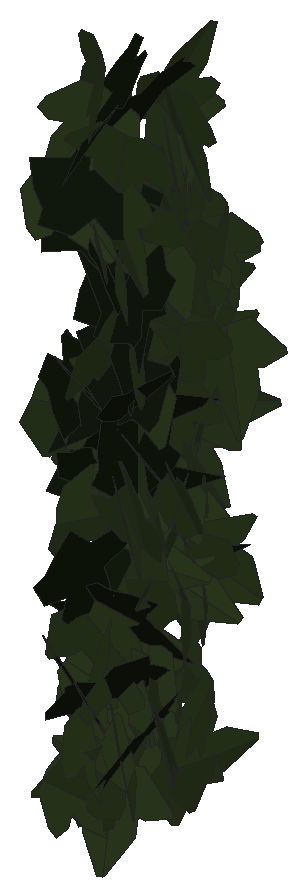
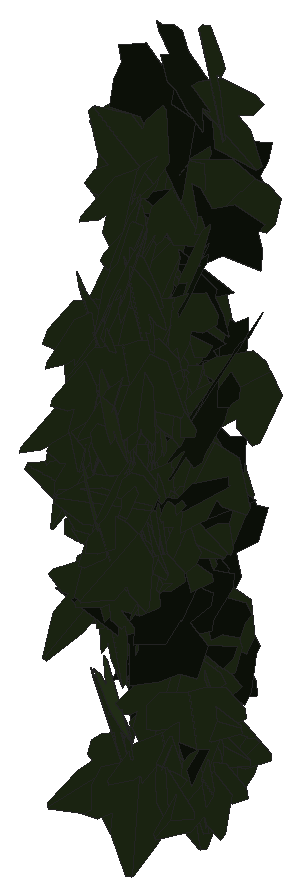
# SketchUp Ruby script. Lengths in inches.
U = 1.inch
M = Sketchup.active_model
def pt(a) = Geom::Point3d.new(a.map { |v| v * U })
def face(e, loops, mat)
  f = e.add_face(loops[0].map { |a| pt(a) })
  loops[1..].each { |l| e.add_face(l.map { |a| pt(a) }).erase! }
  f.material = f.back_material = mat if mat
  f
end
# faces: each face lists its corners as indices into pts; further lists are holes
def faces(e, pts, list, mat = nil) = list.each { |f| face(e, (f[0].is_a?(Array) ? f : [f]).map { |l| l.map { |i| pts[i] } }, mat) }
# xy, xz, yz: faces in a plane at the given z, y or x. An outline is a flat list of corners, or four numbers for a rectangle; further outlines are holes
def ring(l) = l.size == 4 ? [[l[0], l[1]], [l[2], l[1]], [l[2], l[3]], [l[0], l[3]]] : l.each_slice(2).to_a
def flat(e, list, mat, &to3) = list.each { |f| face(e, (f[0].is_a?(Array) ? f : [f]).map { |l| ring(l).map { |u, v| to3.(u, v) } }, mat) }
def xy(e, z, list, mat = nil) = flat(e, list, mat) { |x, y| [x, y, z] }
def xz(e, y, list, mat = nil) = flat(e, list, mat) { |x, z| [x, y, z] }
def yz(e, x, list, mat = nil) = flat(e, list, mat) { |y, z| [x, y, z] }
def lines(e, pts, list) = list.each { |a, b| e.add_line(pt(pts[a]), pt(pts[b])) }
# prism: a flat outline (further loops are holes) pulled along v
def prism(e, loops, v, mat = nil)
  f = face(e, loops, mat); d = Geom::Vector3d.new(v.map { |x| x * U })
  f.pushpull(f.normal.samedirection?(d) ? d.length : -d.length)
end
def box(e, o, s, mat = nil) = prism(e, [[o, [o[0] + s[0], o[1], o[2]], [o[0] + s[0], o[1] + s[1], o[2]], [o[0], o[1] + s[1], o[2]]]], [0, 0, s[2]], mat)
def at(x, y, z, deg = 0) = Geom::Transformation.translation(pt([x, y, z])) * Geom::Transformation.rotation(ORIGIN, Z_AXIS, deg.degrees)
def axes(o, x, y, z) = Geom::Transformation.new([*x, 0, *y, 0, *z, 0, *pt(o).to_a, 1])
def part(name) = M.definitions.add(name)
# library, detail: a bought-in or finely detailed component or shape, given as its bounding box
def library(name, o, s) = part(name).tap { |d| box(d.entities, o, s) }
def detail(e, o, s) = box(e.add_group.entities, o, s)
def put(e, d, t, mat = nil) = e.add_instance(d, t).tap { |i| i.material = mat if mat }
def group(e, t, mat = nil) = e.add_group.tap { |g| g.transformation = t; g.material = mat if mat }.entities
root = M.entities
M.materials.add("efeu1").color = [18, 25, 13]
M.materials.add("efeu2").color = [43, 57, 29]
c1 = part("ivyleaf_9")
p = [[1.54,2.16,1.25],[1.36,2.04,1.19],[-0.21,0.99,0.68],[-0.71,1.11,0.82],[-0.85,0.86,0.67],[-0.8,0.17,0.21],
  [-0.9,-0.01,0.1],[-0.67,-0.16,-0.02],[-0.08,-0.08,-0.05],[-0.03,-0.6,-0.4],[0.65,-0.88,-0.66],[0.83,-0.6,-0.49],
  [1.29,-0.42,-0.43],[1.8125,-0.07,-0.26],[1.21,0.44,0.15]]
faces(c1.entities,p,[[0,1,2,3,4,5,6,7,8,9,10,11,12,13,14]],"efeu1")
c2 = part("ivyleaf_10")
p = [[0,0.5,-0.03],[-0.0625,2.02,-0.43],[-0.19,2.01,-0.46],[-0.54,1.05,-0.29],[-0.52,0.625,-0.18],[-0.83,0.76,-0.28],
  [-1.16,0.64,-0.33],[-1.15,0.33,-0.24],[-0.77,-0.39,0.02],[-0.3,-0.51,0.16],[0.04,-0.48,0.23],[-0.02,2.01,-0.4375],
  [-0.06,2.01,-0.43],[0.04,-0.49,0.23],[0.67,-0.49,0.14],[1.38,0.36,-0.2],[1.375,0.51,-0.24],[0.81,0.65,-0.19],
  [0.62,0.59,-0.15],[0.6,1.09,-0.28],[0.5,1.23,-0.31]]
faces(c2.entities,p,[[0,1,2,3,4,5,6,7,8,9,10],[11,12,0,13,14,15,16,17,18,19,20]],"efeu2")
put(root,c1,axes([53.375,224.15,219.1],[0.426,-0.23373,0.11786],[0.10111,-0.06073,-0.48589],[0.24145,0.43781,-0.00448]))
put(root,c2,axes([54.18,224.19,217.5],[-0.491,0.09443,0.00209],[-0.00146,-0.01868,0.49965],[0.09445,0.49065,0.01862]))
put(root,c2,axes([53.87,224.28,221.39],[-0.32755,0.13032,-0.35458],[0.25629,-0.26811,-0.33531],[-0.27753,-0.40141,0.10884]))
put(root,c1,axes([53.33,224.05,219.33],[0.3048,-0.29469,-0.26506],[-0.16601,0.20871,-0.42294],[0.35991,0.34583,0.02938]))
put(root,c1,axes([53.31,224.02,215.61],[0.4394,-0.07762,-0.22562],[-0.2213,0.04415,-0.44618],[0.08919,0.49196,0.00445]))
put(root,c2,axes([54.05,224.11,218.01],[-0.24749,0.43273,-0.03862],[0.01845,-0.03394,-0.49851],[-0.43406,-0.24818,0.00083]))
put(root,c1,axes([54.14,224.34,219.53],[-0.49573,-0.06279,0.01772],[-0.01756,-0.00242,-0.49969],[0.06284,-0.49604,0.00019]))
put(root,c1,axes([53.74,224.03,221.39],[-0.37814,-0.0703,0.31948],[0.32005,0.02152,0.38354],[-0.06768,0.49457,0.02872]))
put(root,c2,axes([54.05,224.17,222.22],[-0.45593,-0.16191,0.12614],[-0.11682,-0.04794,-0.48379],[0.16876,-0.47062,0.00589]))
put(root,c2,axes([53.625,224.27,222.46],[0.41306,0.10684,-0.2607],[-0.25078,-0.07142,-0.42662],[-0.12839,0.4832,-0.00541]))
put(root,c1,axes([53.53,223.86,216.68],[0.04097,-0.02671,0.4976],[0.34876,0.35815,-0.00949],[-0.35593,0.34787,0.04798]))
put(root,c2,axes([53.92,224.13,214.375],[0.07806,0.08591,0.48634],[-0.49367,-0.00032,0.07929],[0.01394,-0.49256,0.08478]))
put(root,c2,axes([53.21,223.96,218.92],[-0.11739,-0.15802,-0.45962],[0.34996,0.30063,-0.19274],[0.33727,-0.36695,0.04002]))
put(root,c2,axes([53.55,224.22,214.41],[-0.23664,-0.43832,-0.04334],[0.0265,0.03494,-0.49807],[0.43966,-0.23802,0.0067]))
put(root,c2,axes([53.55,224.1875,215.31],[0.36373,-0.3388,0.054],[-0.02742,0.04974,0.49676],[-0.34197,-0.36434,0.0176]))
put(root,c1,axes([54.26,224.1875,215.04],[-0.20667,0.44507,-0.09591],[0.04148,-0.08649,-0.49071],[-0.45339,-0.21079,-0.00117]))
put(root,c2,axes([53.5,223.93,217.57],[-0.04536,-0.10795,-0.4861],[0.20831,0.43923,-0.11698],[0.45227,-0.21313,0.00513]))
put(root,c2,axes([53.66,224.13,223.03],[0.25478,-0.27483,-0.33099],[-0.18689,0.27578,-0.37285],[0.3875,0.31371,0.0378]))
put(root,c1,axes([53.86,224.5,223.04],[-0.37347,0.08581,-0.32118],[0.26972,-0.20417,-0.36819],[-0.19434,-0.44827,0.10621]))
put(root,c2,axes([53.15,224.16,221.48],[0.32418,0.21688,0.31285],[0.25262,0.18483,-0.3899],[-0.28477,0.41086,0.01026]))
put(root,c2,axes([53.8,224.09,219.77],[-0.09208,-0.37712,-0.31512],[0.0622,0.30908,-0.38807],[0.4875,-0.11067,-0.01001]))
put(root,c2,axes([53.66,224.36,218.48],[0.31314,-0.00489,0.38977],[0.38971,-0.0067,-0.31318],[0.00828,0.49993,-0.00038]))
put(root,c2,axes([53.375,224.07,214.27],[0.10339,0.40522,0.27406],[0.05674,0.26829,-0.41809],[-0.48589,0.11756,0.00949]))
put(root,c1,axes([54.08,223.92,218.96],[0.24016,0.26598,0.34868],[0.20896,0.28011,-0.35759],[-0.38556,0.31748,0.02339]))
put(root,c2,axes([53.56,224.24,214.87],[0.09736,0.48743,0.05416],[0.00845,0.05354,-0.49705],[-0.49036,0.09771,0.00219]))
put(root,c2,axes([53.69,224.26,218.94],[0.21538,0.44611,0.06782],[0.02851,0.06155,-0.49538],[-0.45033,0.21726,0.00107]))
put(root,c1,axes([53.79,224.45,220.39],[-0.3053,-0.10291,-0.38236],[0.36528,0.11316,-0.32212],[0.15283,-0.47603,0.00609]))
put(root,c2,axes([54.15,224.36,219.28],[0.36402,-0.01789,-0.3423],[-0.339,0.05509,-0.36338],[0.05072,0.49663,0.02798]))
put(root,c2,axes([53.5,224.26,216.2],[-0.34831,-0.24453,-0.26246],[0.24067,0.11197,-0.42372],[0.266,-0.42151,0.0397]))
put(root,c1,axes([54.16,224.14,218.26],[-0.08789,-0.17612,0.45963],[0.29016,0.35861,0.19289],[-0.3976,0.30063,0.03917]))
put(root,c1,axes([53.7,224.19,215.47],[0.13865,0.47364,-0.08026],[-0.03007,-0.07482,-0.49346],[-0.47945,0.14167,0.00773]))
put(root,c1,axes([54.16,224.27,220.27],[-0.12744,0.17157,0.45202],[-0.33387,0.30688,-0.2106],[-0.3497,-0.35551,0.03635]))
put(root,c2,axes([53.62,224.46,214.0625],[0.43809,0.24051,-0.01524],[-0.01835,0.00175,-0.49966],[-0.2403,0.43835,0.01036]))
put(root,c2,axes([53.74,224.46,214.83],[-0.21612,0.43023,-0.13489],[0.06007,-0.12077,-0.48146],[-0.44686,-0.22431,0.00051]))
put(root,c2,axes([54.16,224.34,219.67],[-0.15599,0.47034,0.06668],[-0.02003,0.06361,-0.49553],[-0.47462,-0.15727,-0.00101]))
put(root,c2,axes([54.3,224.51,220.85],[0.41066,-0.01514,-0.28483],[-0.28307,0.0397,-0.41023],[0.03504,0.49819,0.02404]))
put(root,c1,axes([53.34,224.49,221.28],[-0.17824,-0.21587,-0.41429],[0.28218,0.30363,-0.27961],[0.3723,-0.33348,0.01359]))
put(root,c2,axes([54.27,224.45,216.84],[-0.16494,0.04552,0.46981],[-0.47197,-0.00911,-0.16481],[-0.00644,-0.49784,0.04597]))
put(root,c2,axes([54.35,224.37,215.22],[-0.34848,0.33469,0.12863],[-0.09958,0.08198,-0.48308],[-0.34445,-0.3623,0.00952]))
put(root,c2,axes([54.0625,224.47,221.25],[-0.49968,-0.01522,0.00944],[-0.00936,-0.00255,-0.49991],[0.01526,-0.49976,0.00226]))
put(root,c2,axes([53.72,224.27,214.13],[-0.03693,0.04581,-0.49653],[-0.29662,0.39819,0.05879],[0.40081,0.2989,-0.00223]))
put(root,c1,axes([53.42,224.3,216.3],[0.45878,0.16451,0.11161],[0.10396,0.04075,-0.48737],[-0.16945,0.4704,0.00318]))
put(root,c2,axes([53.38,224.47,215.4375],[0.34763,0.1128,0.34122],[0.30912,0.14829,-0.36394],[-0.1833,0.46399,0.03336]))
put(root,c1,axes([53.41,224.35,217.76],[0.23471,0.0468,0.439],[0.43284,0.07353,-0.23926],[-0.08696,0.49234,-0.006]))
put(root,c2,axes([53.81,224.57,214.86],[0.10614,0.03451,0.48739],[-0.48201,-0.07427,0.11023],[0.08001,-0.49325,0.0175]))
put(root,c1,axes([53.37,224.87,218.42],[0.39345,-0.29135,-0.10157],[0.0817,-0.06034,0.48957],[-0.29753,-0.40184,0.00012]))
put(root,c2,axes([53.55,224.93,218.86],[0.00971,-0.34168,-0.36491],[0.05765,-0.36178,0.34028],[-0.49657,-0.04869,0.03237]))
put(root,c1,axes([54.05,224.45,222.78],[-0.06676,0.49365,-0.04309],[-0.00502,-0.04415,-0.49802],[-0.4955,-0.06607,0.01085]))
put(root,c2,axes([53.46,224.52,220.84],[-0.23649,0.42577,0.11311],[-0.06798,0.09157,-0.48682],[-0.43526,-0.24564,0.01458]))
put(root,c2,axes([53.49,225,214.42],[0.04346,-0.28328,0.40971],[0.17584,-0.37606,-0.27867],[0.46604,0.16831,0.06693]))
put(root,c1,axes([53.4375,224.57,220.64],[0.37442,-0.23066,-0.23793],[-0.19152,0.14234,-0.43938],[0.27043,0.42016,0.01824]))
put(root,c2,axes([53.67,224.53,216.9375],[-0.10704,-0.15072,-0.46457],[0.43981,0.17707,-0.15878],[0.21239,-0.44264,0.09467]))
put(root,c2,axes([53.32,224.65,218.1875],[-0.43932,-0.16018,-0.17704],[0.17278,0.04256,-0.46726],[0.16476,-0.47173,0.01796]))
put(root,c2,axes([53.51,224.87,221.5625],[0.05052,0.42784,-0.25376],[-0.08982,-0.24303,-0.42763],[-0.48927,0.08879,0.0523]))
put(root,c2,axes([53.46,224.59,215.58],[0.39547,0.27631,-0.13139],[0.106,0.07768,0.48242],[0.287,-0.40941,0.00286]))
put(root,c2,axes([53.7,224.8,215.55],[0.46179,0.06283,-0.18112],[-0.17972,-0.02254,-0.46604],[-0.06673,0.49552,0.00177]))
put(root,c1,axes([53.42,224.9375,217.81],[-0.17819,-0.45169,-0.11926],[0.04586,0.11011,-0.48556],[0.46491,-0.18399,0.00218]))
put(root,c2,axes([53.45,224.5625,217.55],[-0.10123,-0.35886,-0.33313],[0.08482,0.32217,-0.37284],[0.48224,-0.132,-0.00435]))
put(root,c2,axes([53.35,224.46,214.15],[-0.05742,-0.17787,-0.46375],[0.1119,0.45021,-0.18653],[0.48392,-0.12521,-0.0119]))
put(root,c2,axes([53.65,224.72,219.87],[-0.21142,0.4528,0.0167],[-0.0054,0.01591,-0.49972],[-0.45307,-0.21148,-0.00183]))
put(root,c2,axes([53.33,224.83,215.22],[0.37237,0.33115,-0.041],[-0.0305,-0.0274,-0.49832],[-0.33229,0.37361,-0.0002]))
put(root,c2,axes([54.39,224.75,217.57],[-0.36819,0.17786,-0.28775],[-0.26189,0.11934,0.40887],[0.21412,0.4518,0.00528]))
put(root,c2,axes([53.82,224.56,220.48],[-0.12081,0.40113,0.27295],[-0.09163,0.25736,-0.41877],[-0.47645,-0.1512,0.01133]))
put(root,c2,axes([53.96,224.9375,217.45],[0.21194,0.07819,-0.44606],[-0.43398,-0.10565,-0.22473],[-0.12939,0.48242,0.02309]))
put(root,c2,axes([54.03,225.17,216.84],[-0.04938,0.14392,-0.47629],[-0.03203,-0.47855,-0.14128],[-0.49652,0.01656,0.05648]))
put(root,c2,axes([53.78,225.01,218.1],[-0.09248,0.40339,-0.28058],[0.02502,-0.28127,-0.41263],[-0.49073,-0.09037,0.03184]))
put(root,c1,axes([53.37,224.99,216.43],[0.2831,0.28841,0.2944],[-0.24552,-0.16885,0.40151],[0.33102,-0.3719,0.04602]))
put(root,c2,axes([53.52,224.95,218.11],[0.14286,0.46827,-0.10156],[-0.04656,-0.0919,-0.48927],[-0.47689,0.14925,0.01735]))
put(root,c2,axes([53.77,225,217.21],[-0.28864,0.35721,-0.1977],[0.09706,-0.17514,-0.45815],[-0.39657,-0.30286,0.03176]))
put(root,c2,axes([53.58,225.02,214.72],[0.20867,0.4375,-0.12267],[-0.04425,-0.11478,-0.48463],[-0.45222,0.21311,-0.00918]))
put(root,c2,axes([54.01,224.9375,218.83],[-0.46223,-0.1904,0.0095],[-0.01042,0.00035,-0.49989],[0.19036,-0.46233,-0.00429]))
put(root,c2,axes([54.16,224.95,219.54],[-0.33893,-0.36485,-0.04487],[0.02703,0.03613,-0.49796],[0.3666,-0.33997,-0.00477]))
put(root,c2,axes([53.55,225.1875,217.24],[-0.01256,-0.46099,-0.19322],[-0.0072,-0.19309,0.46116],[-0.49979,0.01437,-0.00179]))
put(root,c2,axes([54.02,225.04,217.72],[0.42255,-0.02134,-0.26645],[-0.26614,0.01276,-0.42309],[0.02486,0.49938,-0.00058]))
put(root,c2,axes([53.9,224.91,218.01],[0.29724,-0.30811,-0.25829],[-0.16053,0.20355,-0.42755],[0.36861,0.3371,0.02209]))
put(root,c2,axes([53.61,224.92,215.44],[0.11067,0.48459,0.05404],[0.0128,0.05251,-0.49707],[-0.48743,0.1114,-0.00078]))
put(root,c2,axes([53.75,225.11,216.84],[-0.32053,-0.36626,0.11454],[-0.07551,-0.08612,-0.4867],[0.37625,-0.3293,-0.0001]))
put(root,c2,axes([53.9,224.97,216.63],[-0.20066,-0.23019,-0.39591],[0.41256,0.0968,-0.26538],[0.19882,-0.43318,0.15108]))
put(root,c2,axes([53.44,225.05,220.23],[0.28334,0.4114,0.02178],[0.0119,0.01825,-0.49953],[-0.4118,0.28358,0.00055]))
put(root,c2,axes([53.875,224.8125,218.89],[0.23336,0.00673,0.44215],[-0.34654,0.31333,0.17814],[-0.27468,-0.38959,0.1509]))
put(root,c2,axes([54.32,225.125,215.12],[0.37524,-0.3096,-0.11553],[-0.08993,0.07253,-0.48647],[0.31798,0.38586,-0.00125]))
put(root,c2,axes([54.28,224.84,216.4],[0.16751,-0.06425,-0.4667],[-0.26436,0.39717,-0.14956],[0.38994,0.29687,0.09909]))
put(root,c2,axes([54.01,225.14,217.79],[0.33303,-0.36392,-0.08158],[-0.05645,0.05892,-0.4933],[0.36865,0.33778,-0.00184]))
put(root,c2,axes([53.78,225.27,218.73],[0.02021,0.41744,-0.27447],[-0.09697,-0.26619,-0.41199],[-0.49009,0.06988,0.0702]))
put(root,c2,axes([54.12,225.18,216.86],[-0.37879,-0.31224,0.09497],[-0.0749,-0.05845,-0.49089],[0.31766,-0.38612,-0.0025]))
put(root,c2,axes([53.76,224.8,218.97],[0.11484,0.00671,-0.48659],[-0.08847,0.49191,-0.0141],[0.47852,0.08933,0.11417]))
put(root,c2,axes([54.01,225.18,222.25],[-0.39878,0.23417,-0.19009],[0.14853,-0.12179,-0.46163],[-0.26251,-0.42465,0.02757]))
put(root,c2,axes([54.02,225.05,217.38],[-0.05032,0.01353,0.49728],[-0.4795,0.13179,-0.0521],[-0.13249,-0.48213,-0.00029]))
put(root,c1,axes([53.32,224.98,216.34],[0.18199,0.35865,-0.29707],[0.13826,0.26295,0.40217],[0.4447,-0.22853,-0.00346]))
put(root,c2,axes([53.8,225.22,214.21],[-0.46474,-0.18272,0.02521],[-0.0222,-0.01241,-0.49935],[0.18311,-0.46525,0.00342]))
put(root,c2,axes([54.06,225.1875,220.45],[-0.01946,-0.45749,-0.2008],[0.11624,0.19129,-0.44709],[0.48591,-0.06408,0.09892]))
put(root,c2,axes([54.05,225.21,217.94],[-0.38335,0.19837,0.25238],[-0.26583,0.02419,-0.42279],[-0.17995,-0.45833,0.08692]))
put(root,c2,axes([53.71,225.61,215.2],[-0.02223,-0.17475,-0.46794],[0.27429,-0.39573,0.13475],[-0.41746,-0.25071,0.11346]))
put(root,c2,axes([53.81,225.21,219.8125],[-0.34306,-0.27788,-0.23471],[0.17604,0.15549,-0.4414],[0.3183,-0.38549,-0.00885]))
put(root,c2,axes([53.57,225.14,217.22],[0.08806,-0.36512,0.33005],[-0.08714,0.31843,0.37552],[-0.48441,-0.12365,-0.00755]))
put(root,c2,axes([54.17,225.11,214.28],[-0.03073,-0.06539,-0.49475],[0.17152,0.46411,-0.07199],[0.46865,-0.17415,-0.00609]))
put(root,c2,axes([54.11,225.27,216.43],[0.27633,-0.12234,-0.39834],[-0.22901,0.35473,-0.26781],[0.34814,0.33046,0.14]))
put(root,c2,axes([53.55,225.54,217.07],[0.27654,0.41262,-0.05715],[-0.0291,-0.04929,-0.49671],[-0.41554,0.27805,-0.00325]))
put(root,c2,axes([53.625,225.4,222.125],[-0.05162,-0.43992,0.23195],[0.01825,0.23137,0.44287],[-0.49699,0.05419,-0.00783]))
put(root,c2,axes([53.46,225.62,221.33],[-0.23948,0.40031,-0.18001],[0.08613,-0.15821,-0.46642],[-0.43039,-0.2544,0.00682]))
put(root,c2,axes([53.61,225.54,221.99],[0.04102,0.49821,0.01025],[0.00178,0.01014,-0.49989],[-0.49831,0.04105,-0.00094]))
put(root,c2,axes([53.57,225.82,220.4],[-0.13937,0.37051,0.30545],[0.1081,-0.28568,0.39586],[0.46786,0.17638,-0.00048]))
put(root,c2,axes([53.58,225.58,221.59],[-0.23104,0.44238,-0.03037],[-0.00984,-0.03935,-0.49835],[-0.44331,-0.22968,0.02689]))
put(root,c2,axes([53.48,225.67,221.08],[0.41272,-0.27029,-0.08126],[-0.04772,0.07505,-0.49203],[0.27818,0.41389,0.03616]))
put(root,c2,axes([54.16,225.36,216.68],[0.08686,0.32769,0.36753],[0.02874,0.36919,-0.33596],[-0.49156,0.07949,0.0453]))
put(root,c2,axes([53.46,225.63,221.2],[-0.17715,0.46537,-0.04526],[0.00869,-0.04512,-0.49788],[-0.46748,-0.17719,0.0079]))
put(root,c2,axes([53.36,225.8125,221.02],[0.43815,-0.21359,0.11138],[0.10356,-0.04173,-0.48738],[0.21749,0.45015,0.00767]))
put(root,c2,axes([53.45,225.71,219.55],[-0.45351,0.19618,-0.07643],[0.0485,-0.07929,-0.49129],[-0.20488,-0.45302,0.05289]))
put(root,c2,axes([53.49,225.87,218.85],[0.14319,-0.4679,-0.1028],[0.02838,-0.09882,0.48932],[-0.47822,-0.14596,-0.00174]))
put(root,c2,axes([53.47,225.8,219.95],[0.35326,0.34898,-0.05852],[-0.04851,-0.03415,-0.49647],[-0.35051,0.35644,0.00973]))
put(root,c2,axes([53.43,225.76,219.79],[-0.44897,-0.18162,-0.12425],[0.13242,0.00248,-0.48214],[0.17575,-0.46584,0.04587]))
put(root,c2,axes([53.59,225.91,219.6],[0.17759,-0.46314,0.06297],[0.0285,-0.05651,-0.49598],[0.46653,0.17976,0.00633]))
put(root,c2,axes([53.92,225.89,220.52],[0.38869,-0.31397,-0.01845],[-0.01436,0.01159,-0.49966],[0.31419,0.38896,-0.00001]))
put(root,c2,axes([53.49,225.85,218.52],[-0.15542,0.45992,-0.11966],[0.04607,-0.11072,-0.48541],[-0.47299,-0.16191,-0.00796]))
put(root,c2,axes([53.87,225.84,220.26],[0.06576,0.49368,-0.04427],[-0.05813,-0.03667,-0.49525],[-0.49224,0.07028,0.05257]))
put(root,c2,axes([53.54,225.64,221.28],[-0.14898,0.38364,0.28395],[-0.09732,0.26679,-0.41152],[-0.46726,-0.17789,-0.00483]))
put(root,c2,axes([53.78,225.84,220.3],[-0.36428,-0.31003,-0.14554],[0.13579,0.06432,-0.47689],[0.31442,-0.38697,0.03733]))
put(root,c2,axes([54.15,225.87,219.04],[0.08915,0.4919,-0.0093],[-0.00006,-0.00944,-0.49991],[-0.49199,0.08914,-0.00162]))
put(root,c2,axes([53.62,225.86,219.46],[-0.13415,0.48125,0.02002],[-0.00502,0.01939,-0.4996],[-0.48164,-0.13424,-0.00037]))
put(root,c2,axes([53.76,226.05,218.47],[0.24741,-0.43434,0.01159],[0.00891,-0.00826,-0.49985],[0.43441,0.24755,0.00365]))
put(root,c2,axes([53.32,226.05,217.74],[-0.42022,0.04712,-0.26682],[0.25705,-0.08634,-0.42008],[-0.08566,-0.49023,0.04834]))
put(root,c2,axes([53.6,225.97,218.12],[-0.13007,-0.1286,0.46534],[0.42612,0.19597,0.17326],[-0.22695,0.44165,0.05862]))
put(root,c2,axes([53.8,225.89,219.6],[0.00344,0.46411,0.18598],[-0.11602,0.18165,-0.45115],[-0.48634,-0.04005,0.10895]))
put(root,c2,axes([53.42,225.82,218.11],[0.01849,-0.22918,0.444],[0.04095,0.4435,0.22722],[-0.49798,0.02797,0.03517]))
put(root,c2,axes([53.4375,225.83,217.98],[0.15476,0.1981,-0.43221],[0.26807,0.33904,0.25138],[0.39267,-0.30953,-0.00127]))
put(root,c2,axes([53.77,225.96,218.83],[0.01865,0.39824,0.30176],[-0.02984,0.30232,-0.39713],[-0.49876,-0.0032,0.03505]))
